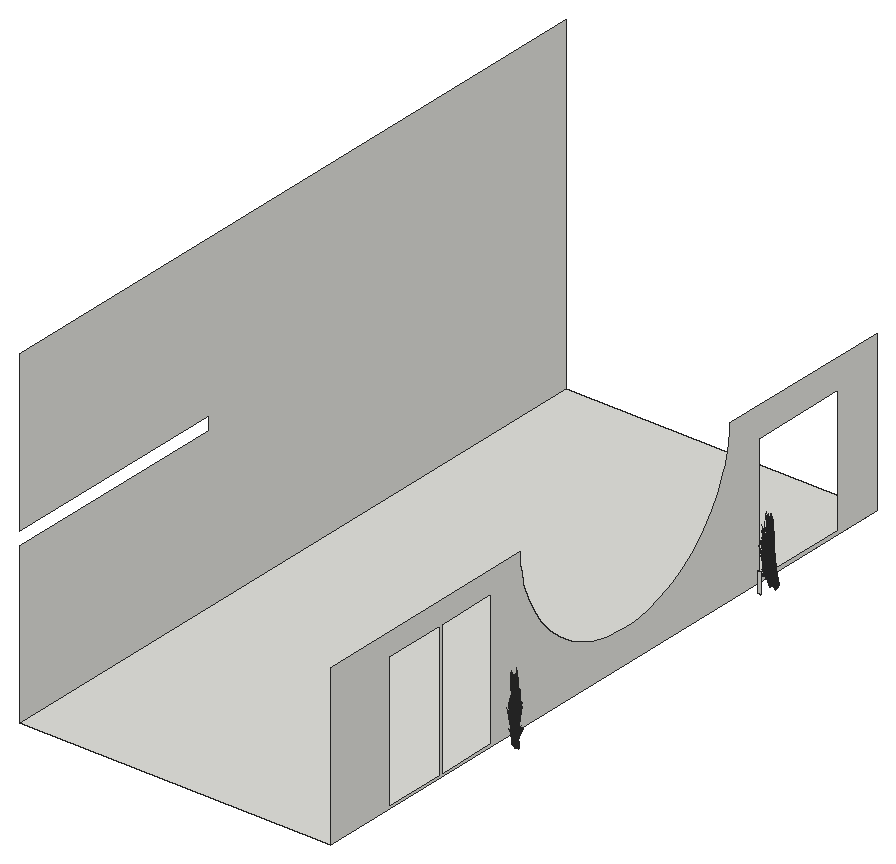
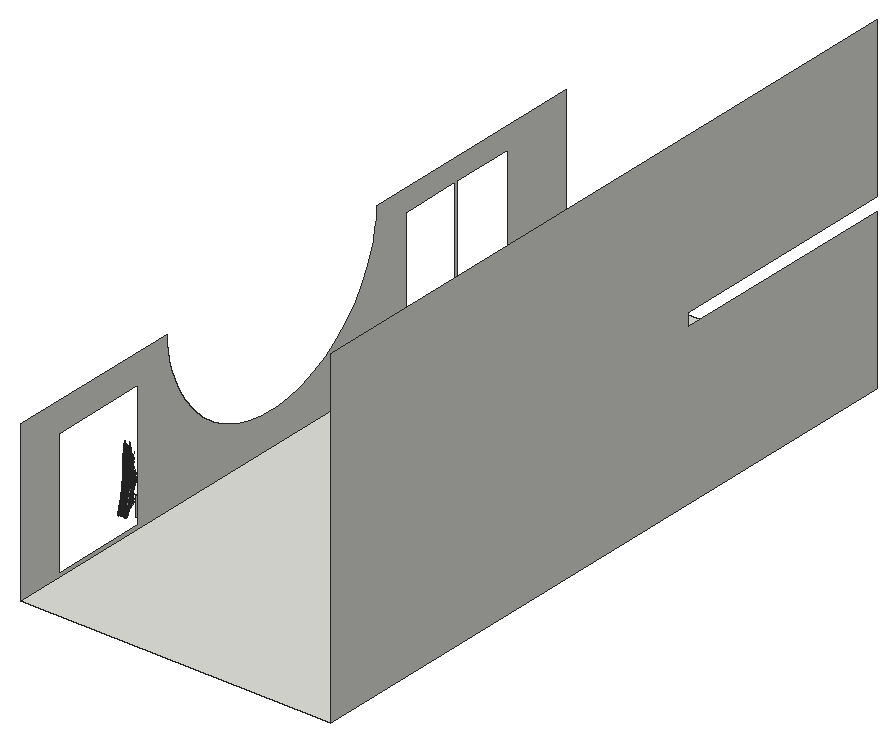
# SketchUp Ruby script. Lengths in inches.
U = 1.inch
M = Sketchup.active_model
def pt(a) = Geom::Point3d.new(a.map { |v| v * U })
def face(e, loops, mat)
  f = e.add_face(loops[0].map { |a| pt(a) })
  loops[1..].each { |l| e.add_face(l.map { |a| pt(a) }).erase! }
  f.material = f.back_material = mat if mat
  f
end
# faces: each face lists its corners as indices into pts; further lists are holes
def faces(e, pts, list, mat = nil) = list.each { |f| face(e, (f[0].is_a?(Array) ? f : [f]).map { |l| l.map { |i| pts[i] } }, mat) }
# xy, xz, yz: faces in a plane at the given z, y or x. An outline is a flat list of corners, or four numbers for a rectangle; further outlines are holes
def ring(l) = l.size == 4 ? [[l[0], l[1]], [l[2], l[1]], [l[2], l[3]], [l[0], l[3]]] : l.each_slice(2).to_a
def flat(e, list, mat, &to3) = list.each { |f| face(e, (f[0].is_a?(Array) ? f : [f]).map { |l| ring(l).map { |u, v| to3.(u, v) } }, mat) }
def xy(e, z, list, mat = nil) = flat(e, list, mat) { |x, y| [x, y, z] }
def xz(e, y, list, mat = nil) = flat(e, list, mat) { |x, z| [x, y, z] }
def yz(e, x, list, mat = nil) = flat(e, list, mat) { |y, z| [x, y, z] }
def lines(e, pts, list) = list.each { |a, b| e.add_line(pt(pts[a]), pt(pts[b])) }
# prism: a flat outline (further loops are holes) pulled along v
def prism(e, loops, v, mat = nil)
  f = face(e, loops, mat); d = Geom::Vector3d.new(v.map { |x| x * U })
  f.pushpull(f.normal.samedirection?(d) ? d.length : -d.length)
end
def box(e, o, s, mat = nil) = prism(e, [[o, [o[0] + s[0], o[1], o[2]], [o[0] + s[0], o[1] + s[1], o[2]], [o[0], o[1] + s[1], o[2]]]], [0, 0, s[2]], mat)
def at(x, y, z, deg = 0) = Geom::Transformation.translation(pt([x, y, z])) * Geom::Transformation.rotation(ORIGIN, Z_AXIS, deg.degrees)
def axes(o, x, y, z) = Geom::Transformation.new([*x, 0, *y, 0, *z, 0, *pt(o).to_a, 1])
def part(name) = M.definitions.add(name)
# library, detail: a bought-in or finely detailed component or shape, given as its bounding box
def library(name, o, s) = part(name).tap { |d| box(d.entities, o, s) }
def detail(e, o, s) = box(e.add_group.entities, o, s)
def put(e, d, t, mat = nil) = e.add_instance(d, t).tap { |i| i.material = mat if mat }
def group(e, t, mat = nil) = e.add_group.tap { |g| g.transformation = t; g.material = mat if mat }.entities
root = M.entities
M.materials.add("LightPink_Translucent").color = [144, 107, 117]
M.materials["LightPink_Translucent"].alpha = 0.75
c1 = part("blade")
p = [[2.15,0.21,22],[0,0.17,0],[0.09,0.45,0],[2.18,0.31,22],[2.29,0.31,22],[0.38,0.45,0],
  [2.48,0.24,33],[2.49,0.24,33],[2.48,0.22,33]]
faces(c1.entities,p,[[0,1,2,3],[4,5,2,3],[6,3,4,7],[8,0,3,6]])
c2 = part("seeds")
p = [[0.3,-0.1,1.38],[-0.01,-0.03,1.59],[-0.01,-0.03,0.03],[0.14,-0.07,-0.07],[0.29,-0.03,3],[0.15,0.01,3.11]]
faces(c2.entities,p,[[0,1,2,3],[1,0,4,5]],"LightPink_Translucent")
c3 = part("blade with seeds")
put(c3.entities,c1,at(0,0,0))
put(c3.entities,c2,axes([2.4,0.25,30.99],[1.5799,-0.05474,1.17369],[-0.12525,1.92788,0.29478],[-0.07173,-0.02425,1.56792]))
xy(root,618,[[39.57,167.5625,321.57,786.64]])
xz(root,361.54,[[330.57,618,333.57,636]])
xz(root,640.9,[[330.57,618,333.57,636]])
yz(root,39.57,[[167.5625,618,786.64,618,786.64,918,167.5625,918,167.5625,774,381.61,774,381.24,765.87,381.55,762,167.5625,762]])
yz(root,321.57,[[[167.5625,618,167.5625,762,381.51,762,381.51,761.73,382.09,755.37,382.45,750.85,382.53,750.46,382.63,749.39,385.28,737.31,385.54,736.1,385.57,736,385.87,734.67,390.92,720.47,397.71,707.02,406.14,694.53,416.0625,683.1875,427.33,673.18,439.76,664.67,453.17,657.78,467.33,652.62,482.02,649.28,497.02,647.81,501.22,647.92,512.08,648.23,526.98,650.53,541.46,654.68,555.3125,660.62,568.3125,668.24,580.25,677.43,590.95,688.05,600.23,699.93,607.94,712.87,613.98,726.68,614.22,727.97,617.96,740.22,620.52,755.07,620.84,762,786.64,762,786.64,618],[652.9,621,742.9,735],[233.15,620,291.15,742],[293.15,620,349.15,742]]])
put(root,c3,axes([334.28,650.62,623.6],[0.14639,-0.01056,1.71376],[-0.09712,0.45778,0.13857],[-0.20862,-0.02831,0.73262]))
put(root,c3,axes([334.71,650.19,624.71],[-0.35281,-0.01123,-0.71045],[0.0237,-0.47284,0.08574],[-0.14947,-0.0499,1.00501]))
put(root,c3,axes([334.43,650.31,622.31],[0.06891,0.12984,1.43002],[-0.15879,0.35293,-0.30754],[-0.16304,-0.08436,0.61141]))
put(root,c3,axes([334.55,649.89,623.6],[0.1311,0.08035,1.71376],[-0.27131,0.33708,0.13857],[-0.16909,-0.15206,0.73262]))
put(root,c3,axes([334.6,650.29,624.4],[-0.25628,0.30892,-0.51099],[-0.22444,-0.32634,-0.3958],[-0.13021,-0.047,0.97773]))
put(root,c3,axes([334.24,649.42,624.43],[0.02617,0.04654,1.77383],[-0.12614,0.41836,-0.16761],[-0.12775,0.00303,0.31391]))
put(root,c3,axes([334.53,649.15,624.4375],[-0.07594,-0.00329,1.74944],[-0.24177,0.32918,-0.27667],[-0.129,-0.06726,0.14031]))
put(root,c3,axes([334.73,649.97,624.76],[-0.0189,0.47427,-0.1216],[-0.35781,-0.01296,-0.67495],[-0.13781,-0.03295,1.02557]))
put(root,c3,axes([334.5,650,624.25],[-0.20082,-0.29199,-0.35414],[0.2293,-0.2764,0.4572],[-0.1165,-0.04206,0.87481]))
put(root,c3,axes([334.02,650.7,622.49],[0.22533,-0.03337,1.1486],[-0.14293,0.29403,0.84392],[-0.11135,-0.04411,0.25299]))
put(root,c3,axes([334.47,649.89,624.82],[0.29147,-0.34417,0.53763],[0.25138,0.3655,0.4433],[-0.13675,-0.06349,1.11249]))
put(root,c3,axes([334.6,649.89,624.45],[0.01777,-0.35463,0.0643],[0.26836,0.00972,0.50621],[-0.1028,-0.03711,0.77189]))
put(root,c3,axes([335.43,649.27,625.15],[-0.23555,0.44708,-0.13619],[-0.34112,-0.25757,-0.75594],[-0.11858,-0.12631,1.14864]))
put(root,c3,axes([334.79,650.15,624.78],[0.20082,0.29199,0.35414],[-0.2293,0.2764,-0.4572],[-0.1165,-0.04206,0.87481]))
put(root,c3,axes([335.33,649.64,624.71],[-0.30095,-0.22541,-0.71045],[0.21388,-0.395,0.08574],[-0.10904,-0.13459,1.00501]))
put(root,c3,axes([335.1875,649.65,624.4],[-0.34827,0.11086,-0.51099],[-0.06092,-0.41983,-0.3958],[-0.09354,-0.12031,0.97773]))
put(root,c3,axes([334.74,649.27,621.22],[-0.03419,0.06144,1.76342],[-0.3455,0.13246,-0.26939],[-0.08346,-0.12049,0.30037]))
put(root,c3,axes([334.52,649.5,621.85],[-0.10181,0.3808,-0.03893],[-0.31336,-0.11714,-0.17649],[-0.04758,-0.06228,0.58215]))
put(root,c3,axes([336.78,355.32,621.875],[0.12246,-0.09864,1.71376],[0.1031,0.45582,0.13857],[-0.19225,0.10302,0.73262]))
put(root,c3,axes([335.34,648.21,624.43],[-0.00658,0.0559,1.77383],[-0.32474,0.20287,-0.16761],[-0.09556,-0.1037,0.31391]))
put(root,c3,axes([334.99,649.02,622.31],[-0.02137,0.15256,1.43002],[-0.31245,0.12771,-0.30754],[-0.07303,-0.19719,0.61141]))
put(root,c3,axes([336.4,356.1,620.59],[0.12266,0.03828,1.43002],[0.07906,0.39104,-0.30754],[-0.16661,0.0732,0.61141]))
put(root,c3,axes([335.09,649.42,623.6],[0.08068,0.14973,1.71376],[-0.3728,0.12606,0.13857],[-0.08426,-0.23506,0.73262]))
put(root,c3,axes([335.22,649.34,624.25],[-0.05451,-0.37564,-0.35414],[0.31161,-0.09919,0.4572],[-0.0837,-0.10765,0.87481]))
put(root,c3,axes([337.49,354.85,621.34],[0.10032,-0.06746,1.77064],[0.0346,0.47103,0.13857],[-0.2173,0.0625,0.63284]))
put(root,c3,axes([334.35,651.24,622.1],[-0.44133,0,0],[0,-0.52122,-0.51607],[0,-0.11871,1.63711]))
put(root,c3,axes([335.41,649.65,624.78],[0.05451,0.37564,0.35414],[-0.31161,0.09919,-0.4572],[-0.0837,-0.10765,0.87481]))
put(root,c3,axes([336.41,355.16,622.72],[-0.05763,0.06055,1.74944],[0.0049,0.44239,-0.27667],[-0.13211,0.05753,0.14031]))
put(root,c3,axes([334.7,651.1,622.05],[-0.32829,0.39208,0.30756],[-0.32849,-0.38796,-0.36492],[-0.01146,-0.11134,1.64885]))
put(root,c3,axes([336.05,652.1875,623.05],[0.305,0.18805,1.51261],[-0.29879,0.40513,0.59816],[-0.13384,-0.24012,1.26806]))
put(root,c3,axes([334.88,648.78,622.49],[0.18411,0.16231,1.1486],[-0.26813,0.09757,0.84392],[-0.05737,-0.12474,0.25299]))
put(root,c3,axes([335.55,651.7,621.93],[-0.21202,-0.39143,-0.44739],[0.32115,-0.27564,0.21531],[-0.06861,-0.04843,1.43643]))
put(root,c3,axes([335.27,649.2,624.82],[0.39316,-0.11987,0.53763],[0.06823,0.47021,0.4433],[-0.09247,-0.13858,1.11249]))
put(root,c3,axes([335.77,355.61,622.71],[0.04504,0.01251,1.77383],[0.13934,0.41205,-0.16761],[-0.0922,0.10815,0.31391]))
put(root,c3,axes([336.79,355.11,622.68],[-0.09562,0.42421,-0.51099],[-0.32782,-0.1454,-0.3958],[-0.13199,0.0389,0.97773]))
put(root,c3,axes([335.36,649.3,624.45],[0.16041,-0.29625,0.0643],[0.22843,0.17248,0.50621],[-0.07385,-0.09498,0.77189]))
put(root,c3,axes([335.59,651.92,622.16],[0.09355,-0.55261,-0.23429],[0.44354,0.09633,0.51271],[-0.0775,-0.07631,1.5644]))
put(root,c3,axes([336.14,356.92,620.77],[0.14709,-0.21136,1.1486],[0.05804,0.3346,0.84392],[-0.1063,0.05991,0.25299]))
put(root,c3,axes([335.71,648.43,624.4375],[-0.05398,-0.06539,1.74944],[-0.36026,0.04145,-0.27667],[-0.0575,-0.15639,0.14031]))
put(root,c3,axes([334.45,650.89,621.74],[0,-0.46636,-0.49651],[0.39487,0,0],[0,-0.10622,1.57504]))
put(root,c3,axes([334.62,651.32,622.2],[0,0.46636,0.49651],[-0.39487,0,0],[0,-0.10622,1.57504]))
put(root,c3,axes([336.78,354.74,623.03],[0.17758,0.42229,-0.1216],[-0.31518,0.20752,-0.67495],[-0.13282,0.05572,1.02557]))
put(root,c3,axes([337.23,355.63,621.875],[0.08815,-0.14329,1.71376],[0.22258,0.38678,0.13857],[-0.15267,0.17614,0.73262]))
put(root,c3,axes([336.7,356.01,622.53],[-0.30722,0.06665,-0.35414],[-0.08112,-0.381,0.4572],[-0.08804,0.10234,0.87481]))
put(root,c3,axes([336.53,357.14,619.49],[0.04734,0.04659,1.76342],[0.08027,0.4317,-0.26939],[-0.10492,0.09206,0.30037]))
put(root,c3,axes([335.48,651.43,622.39],[-0.39748,-0.22252,-0.29095],[0.19139,-0.46966,-0.50002],[-0.01249,-0.11531,1.59708]))
put(root,c3,axes([336.74,355.92,622.73],[-0.08753,-0.42921,0.48003],[0.34336,-0.07449,0.3958],[-0.1012,0.10094,0.9933]))
put(root,c3,axes([335.31,650.95,621.82],[-0.14494,-0.47823,-0.69835],[0.41752,-0.17223,-0.18329],[-0.01602,-0.16194,1.54149]))
put(root,c3,axes([336.26,649.43,624.76],[-0.34538,0.21713,-0.1216],[-0.16972,-0.38536,-0.67495],[-0.04557,-0.16239,1.02557]))
put(root,c3,axes([335.96,649.45,624.4],[-0.34695,-0.11691,-0.51099],[0.11892,-0.40083,-0.3958],[-0.03181,-0.16138,0.97773]))
put(root,c3,axes([336.67,355.84,622.73],[-0.2423,-0.19613,0.0643],[0.14107,-0.2793,0.50621],[-0.07768,0.0903,0.77189]))
put(root,c3,axes([334.62,650.9,621.75],[0.24637,-0.29097,-0.30978],[0.24637,0.29097,0.30978],[0,-0.09372,1.38974]))
put(root,c3,axes([335.73,649.02,621.85],[-0.2439,0.26754,-0.03893],[-0.22348,-0.29302,-0.17649],[-0.01573,-0.08303,0.58215]))
put(root,c3,axes([337.16,355.98,621.875],[0.06572,-0.16029,1.71376],[0.27569,0.33172,0.13857],[-0.12437,0.20675,0.73262]))
put(root,c3,axes([338.74,650.62,623.1],[0.14639,-0.01056,1.71376],[-0.09712,0.45778,0.13857],[-0.20862,-0.02831,0.73262]))
put(root,c3,axes([336.09,649.53,624.71],[-0.16845,-0.3792,-0.71045],[0.34676,-0.21133,0.08574],[-0.03939,-0.18322,1.00501]))
put(root,c3,axes([336.95,356.05,622.68],[0.09067,0.42583,-0.51099],[-0.34336,0.07449,-0.3958],[-0.0984,0.11438,0.97773]))
put(root,c3,axes([336.42,356.82,622.72],[-0.00877,0.09229,1.74944],[0.24897,0.32105,-0.27667],[-0.06518,0.15182,0.14031]))
put(root,c3,axes([336.15,649.59,624.78],[-0.1064,0.35863,0.35414],[-0.31043,-0.1046,-0.4572],[-0.02846,-0.14439,0.87481]))
put(root,c3,axes([336.79,355.75,623.03],[0.32648,0.25715,-0.1216],[-0.18809,0.3724,-0.67495],[-0.09224,0.12945,1.02557]))
put(root,c3,axes([337.53,356.92,620.375],[-0.22066,0.46731,0],[-0.36918,-0.26061,-0.51607],[-0.08408,-0.05936,1.63711]))
put(root,c3,axes([335.8,648.6875,621.22],[-0.0592,0.0168,1.76342],[-0.32738,-0.18913,-0.26939],[0.00549,-0.15776,0.30037]))
put(root,c3,axes([336.25,356.86,623.65],[0.31145,0.12449,-0.06488],[-0.0958,0.38314,-0.29416],[-0.05094,0.05817,0.97024]))
put(root,c3,axes([336.95,355.78,623.05],[0.30722,-0.06665,0.35414],[0.08112,0.381,-0.4572],[-0.08804,0.10234,0.87481]))
put(root,c3,axes([336.12,649.21,624.25],[0.1064,-0.35863,-0.35414],[0.31043,0.1046,0.4572],[-0.02846,-0.14439,0.87481]))
put(root,c3,axes([335.6,651.14,622.09],[0.15345,0.52148,0.45755],[-0.43845,0.18134,0.17955],[0.00536,-0.09582,1.58856]))
put(root,c3,axes([335.53,651.08,621.93],[0.17124,-0.42022,-0.44739],[0.35581,0.20224,0.21531],[0,-0.09687,1.43643]))
put(root,c3,axes([337.125,357.6,620.59],[0.11138,-0.07357,1.43002],[0.27499,0.22183,-0.30754],[-0.08185,0.19194,0.61141]))
put(root,c3,axes([339.17,650.19,624.21],[-0.35281,-0.01123,-0.71045],[0.0237,-0.47284,0.08574],[-0.14947,-0.0499,1.00501]))
put(root,c3,axes([338.89,650.31,621.81],[0.06891,0.12984,1.43002],[-0.15879,0.35293,-0.30754],[-0.16304,-0.08436,0.61141]))
put(root,c3,axes([339.01,649.89,623.1],[0.1311,0.08035,1.71376],[-0.27131,0.33708,0.13857],[-0.16909,-0.15206,0.73262]))
put(root,c3,axes([337.24,356.79,622.73],[-0.25132,-0.3182,0.48003],[0.2669,-0.27442,0.3958],[-0.04636,0.14929,0.9933]))
put(root,c3,axes([337.15,356.76,622.73],[-0.29004,-0.02173,0.0643],[0.00795,-0.32812,0.50621],[-0.03035,0.12569,0.77189]))
put(root,c3,axes([336.25,649.26,624.45],[0.26007,-0.1585,0.0643],[0.12729,0.28902,0.50621],[-0.02512,-0.1274,0.77189]))
put(root,c3,axes([337.24,356.89,622.53],[-0.23881,0.24554,-0.35414],[-0.22606,-0.28036,0.4572],[-0.0344,0.14245,0.87481]))
put(root,c3,axes([339.8125,650.62,623.19],[0.14639,-0.01056,1.71376],[-0.09712,0.45778,0.13857],[-0.20862,-0.02831,0.73262]))
put(root,c3,axes([336.16,649.29,624.46],[0.34777,0.12192,0.48003],[-0.11892,0.40083,0.3958],[-0.0209,-0.15763,0.9933]))
put(root,c3,axes([335.74,651.29,622.16],[0.39767,0.22603,0.24065],[-0.19139,0.46966,0.50002],[0,-0.10827,1.60543]))
put(root,c3,axes([339.06,650.29,623.9],[-0.25628,0.30892,-0.51099],[-0.22444,-0.32634,-0.3958],[-0.13021,-0.047,0.97773]))
put(root,c3,axes([335.61,650.97,622.44],[-0.38326,0.02879,0.44739],[-0.03466,-0.47788,-0.21531],[0.06861,-0.04843,1.43643]))
put(root,c3,axes([338.46,356.15,620.06],[-0.23773,0.35053,-0.62353],[-0.29532,-0.31785,-0.16365],[-0.09526,0.08744,1.37633]))
put(root,c3,axes([336.39,357.76,622.71],[0.04004,-0.02816,1.77383],[0.33095,0.18728,-0.16761],[-0.00778,0.15594,0.31391]))
put(root,c3,axes([338.7,649.42,623.93],[0.02617,0.04654,1.77383],[-0.12614,0.41836,-0.16761],[-0.12775,0.00303,0.31391]))
put(root,c3,axes([338.99,649.15,623.9375],[-0.07594,-0.00329,1.74944],[-0.24177,0.32918,-0.27667],[-0.129,-0.06726,0.14031]))
put(root,c3,axes([338.625,355.96,620.46],[-0.34464,-0.37536,-0.25192],[0.29,-0.42149,0.5513],[-0.0928,0.04391,1.68216]))
put(root,c3,axes([335.25,649.58,622.1],[-0.22066,-0.46731,0],[0.36918,-0.26061,-0.51607],[0.08408,-0.05936,1.63711]))
put(root,c3,axes([337.4,356.63,623.34],[-0.00918,0.43138,-0.7886],[-0.38672,-0.02897,0.09517],[-0.04081,0.18275,1.11556]))
put(root,c3,axes([339.19,649.97,624.26],[-0.0189,0.47427,-0.1216],[-0.35781,-0.01296,-0.67495],[-0.13781,-0.03295,1.02557]))
put(root,c3,axes([338.96,650,623.75],[-0.20082,-0.29199,-0.35414],[0.2293,-0.2764,0.4572],[-0.1165,-0.04206,0.87481]))
put(root,c3,axes([337.39,357.84,620.77],[-0.00913,-0.2773,1.1486],[0.22824,0.19778,0.84392],[-0.04489,0.13217,0.25299]))
put(root,c3,axes([338.45,355.875,620.21],[-0.38326,0.02879,-0.44739],[-0.03466,-0.47788,0.21531],[-0.06861,0.04843,1.43643]))
put(root,c3,axes([336.17,648.45,622.49],[0.04528,0.27194,1.1486],[-0.25117,-0.15062,0.84392],[0.02703,-0.13924,0.25299]))
put(root,c3,axes([338.48,650.7,621.99],[0.22533,-0.03337,1.1486],[-0.14293,0.29403,0.84392],[-0.11135,-0.04411,0.25299]))
put(root,c3,axes([337.72,356.68,620.48],[0.33032,0.23318,0.49651],[-0.19744,0.41812,0],[-0.07523,-0.05311,1.57504]))
put(root,c3,axes([337.27,357.24,621.36],[0.00775,-0.24075,1.54345],[0.34877,0.12716,0.21329],[-0.03022,0.25658,0.72882]))
put(root,c3,axes([337.25,648.89,624.43],[-0.03584,0.03562,1.77383],[-0.35118,-0.12018,-0.16761],[-0.01271,-0.15545,0.31391]))
put(root,c3,axes([336.97,649.92,624.76],[-0.3879,-0.02311,-0.1216],[0.0106,-0.43749,-0.67495],[0.02694,-0.1685,1.02557]))
put(root,c3,axes([338.93,649.89,624.32],[0.29147,-0.34417,0.53763],[0.25138,0.3655,0.4433],[-0.13675,-0.06349,1.11249]))
put(root,c3,axes([338.85,357.11,620.02],[-0.33032,0.23318,-0.49651],[-0.19744,-0.41812,0],[-0.07523,0.05311,1.57504]))
put(root,c3,axes([338.875,356.98,620.19],[-0.21791,-0.46895,-0.05142],[0.36918,-0.26061,0.51607],[-0.09097,0.04465,1.6363]))
put(root,c3,axes([340.25,650.19,624.3],[-0.35281,-0.01123,-0.71045],[0.0237,-0.47284,0.08574],[-0.14947,-0.0499,1.00501]))
put(root,c3,axes([336.82,649.99,624.78],[-0.23881,0.24554,0.35414],[-0.22606,-0.28036,-0.4572],[0.0344,-0.14245,0.87481]))
put(root,c3,axes([335.68,650.87,622.39],[-0.04113,-0.53214,-0.29095],[0.42835,-0.03218,-0.50002],[0.07543,-0.07088,1.59708]))
put(root,c3,axes([339.97,650.31,621.91],[0.06891,0.12984,1.43002],[-0.15879,0.35293,-0.30754],[-0.16304,-0.08436,0.61141]))
put(root,c3,axes([337.48,356.77,623],[0.25266,0.31335,-0.5672],[-0.2669,0.27442,-0.43934],[-0.03844,0.15921,1.08528]))
put(root,c3,axes([336.71,649.76,624.4],[-0.25266,-0.31335,-0.51099],[0.2669,-0.27442,-0.3958],[0.03844,-0.15921,0.97773]))
put(root,c3,axes([338.78,356.93,620.03],[-0.32928,-0.11539,-0.30978],[0.08291,-0.40636,0.30978],[-0.06638,0.04686,1.38974]))
put(root,c3,axes([337.36,356.54,623.05],[0.23881,-0.24554,0.35414],[0.22606,0.28036,-0.4572],[-0.0344,0.14245,0.87481]))
put(root,c3,axes([340.09,649.89,623.19],[0.1311,0.08035,1.71376],[-0.27131,0.33708,0.13857],[-0.16909,-0.15206,0.73262]))
put(root,c3,axes([338.97,355.1875,620.84],[-0.00964,-0.43909,1.41272],[0.43635,0.11382,0.59816],[-0.1032,0.24027,1.3335]))
put(root,c3,axes([340.46,355.25,621.875],[0.12246,-0.09864,1.71376],[0.1031,0.45582,0.13857],[-0.19225,0.10302,0.73262]))
put(root,c3,axes([340.08,356.02,620.59],[0.12266,0.03828,1.43002],[0.07906,0.39104,-0.30754],[-0.16661,0.0732,0.61141]))
put(root,c3,axes([337.21,356.61,623.4],[0.3879,0.02311,-0.13498],[-0.0106,0.43749,-0.74919],[-0.02694,0.1685,1.13838]))
put(root,c3,axes([339.06,649.89,623.95],[0.01777,-0.35463,0.0643],[0.26836,0.00972,0.50621],[-0.1028,-0.03711,0.77189]))
put(root,c3,axes([335.63,649.69,621.75],[0.32928,0.11539,-0.30978],[-0.08291,0.40636,0.30978],[0.06638,-0.04686,1.38974]))
put(root,c3,axes([337.2,357.24,620.82],[0.32063,-0.08258,0.06507],[0.07371,0.33271,-0.86304],[-0.02033,0.16842,0.7736]))
put(root,c3,axes([338.72,355.75,620.67],[0.04113,0.53214,-0.29095],[-0.42835,0.03218,-0.50002],[-0.07543,0.07088,1.59708]))
put(root,c3,axes([339.89,649.27,624.65],[-0.23555,0.44708,-0.13619],[-0.34112,-0.25757,-0.75594],[-0.11858,-0.12631,1.14864]))
put(root,c3,axes([336.54,649.2,622.31],[-0.10032,0.0944,1.43002],[-0.30046,-0.16522,-0.30754],[0.05569,-0.20547,0.61141]))
put(root,c3,axes([340.13,650.29,624],[-0.25628,0.30892,-0.51099],[-0.22444,-0.32634,-0.3958],[-0.13021,-0.047,0.97773]))
put(root,c3,axes([339.25,650.15,624.28],[0.20082,0.29199,0.35414],[-0.2293,0.2764,-0.4572],[-0.1165,-0.04206,0.87481]))
put(root,c3,axes([337.76,356.32,621.875],[-0.00864,-0.17899,1.71376],[0.37441,0.11874,0.13857],[-0.02316,0.25508,0.73262]))
put(root,c3,axes([339.79,649.64,624.21],[-0.30095,-0.22541,-0.71045],[0.21388,-0.395,0.08574],[-0.10904,-0.13459,1.00501]))
put(root,c3,axes([335.55,649.51,621.74],[0.33032,-0.23318,-0.49651],[0.19744,0.41812,0],[0.07523,-0.05311,1.57504]))
put(root,c3,axes([339.65,649.65,623.9],[-0.34827,0.11086,-0.51099],[-0.06092,-0.41983,-0.3958],[-0.09354,-0.12031,0.97773]))
put(root,c3,axes([339.77,649.42,624.03],[0.02617,0.04654,1.77383],[-0.12614,0.41836,-0.16761],[-0.12775,0.00303,0.31391]))
put(root,c3,axes([341.15,650.62,623.58],[0.14639,-0.01056,1.71376],[-0.09712,0.45778,0.13857],[-0.20862,-0.02831,0.73262]))
put(root,c3,axes([339.2,649.27,620.72],[-0.03419,0.06144,1.76342],[-0.3455,0.13246,-0.26939],[-0.08346,-0.12049,0.30037]))
put(root,c3,axes([340.07,649.15,624.03],[-0.07594,-0.00329,1.74944],[-0.24177,0.32918,-0.27667],[-0.129,-0.06726,0.14031]))
put(root,c3,axes([340.09,355.09,622.72],[-0.05763,0.06055,1.74944],[0.0049,0.44239,-0.27667],[-0.13211,0.05753,0.14031]))
put(root,c3,axes([336.79,649.9,624.71],[0.00918,-0.43138,-0.71045],[0.38672,0.02897,0.08574],[0.04081,-0.18275,1.00501]))
put(root,c3,axes([340.27,649.97,624.35],[-0.0189,0.47427,-0.1216],[-0.35781,-0.01296,-0.67495],[-0.13781,-0.03295,1.02557]))
put(root,c3,axes([340.04,650,623.84],[-0.20082,-0.29199,-0.35414],[0.2293,-0.2764,0.4572],[-0.1165,-0.04206,0.87481]))
put(root,c3,axes([339.56,650.7,622.08],[0.22533,-0.03337,1.1486],[-0.14293,0.29403,0.84392],[-0.11135,-0.04411,0.25299]))
put(root,c3,axes([338.33,356.51,620.2],[-0.35581,-0.20937,0],[0.17124,-0.43505,0],[0,0,1.62707]))
put(root,c3,axes([339.44,355.53,622.71],[0.04504,0.01251,1.77383],[0.13934,0.41205,-0.16761],[-0.0922,0.10815,0.31391]))
put(root,c3,axes([339.15,357.04,620.375],[0.22066,0.46731,0],[-0.36918,0.26061,-0.51607],[-0.08408,0.05936,1.63711]))
put(root,c3,axes([340.47,355.03,622.68],[-0.09562,0.42421,-0.51099],[-0.32782,-0.1454,-0.3958],[-0.13199,0.0389,0.97773]))
put(root,c3,axes([338.98,649.5,621.35],[-0.10181,0.3808,-0.03893],[-0.31336,-0.11714,-0.17649],[-0.04758,-0.06228,0.58215]))
put(root,c3,axes([338.03,357.24,623.0625],[-0.34777,-0.12192,0.53283],[0.11892,-0.40083,0.43934],[0.0209,0.15763,1.10256]))
put(root,c3,axes([336.95,649.64,624.25],[0.23881,-0.24554,-0.35414],[0.22606,0.28036,0.4572],[0.0344,-0.14245,0.87481]))
put(root,c3,axes([337.9375,357.27,622.73],[-0.26007,0.1585,0.0643],[-0.12729,-0.28902,0.50621],[0.02512,0.1274,0.77189]))
put(root,c3,axes([339.8,648.21,623.93],[-0.00658,0.0559,1.77383],[-0.32474,0.20287,-0.16761],[-0.09556,-0.1037,0.31391]))
put(root,c3,axes([337.04,649.77,624.45],[0.29004,0.02173,0.0643],[-0.00795,0.32812,0.50621],[0.03035,-0.12569,0.77189]))
put(root,c3,axes([340.01,649.89,624.41],[0.29147,-0.34417,0.53763],[0.25138,0.3655,0.4433],[-0.13675,-0.06349,1.11249]))
put(root,c3,axes([339.45,649.02,621.81],[-0.02137,0.15256,1.43002],[-0.31245,0.12771,-0.30754],[-0.07303,-0.19719,0.61141]))
put(root,c3,axes([338.8,355.85,620.62],[0.26075,0.2802,0.1448],[-0.2175,0.31612,-0.41347],[-0.06054,0.04274,1.26744]))
put(root,c3,axes([339.55,649.42,623.1],[0.08068,0.14973,1.71376],[-0.3728,0.12606,0.13857],[-0.08426,-0.23506,0.73262]))
put(root,c3,axes([337.33,649.23,624.4375],[-0.00341,-0.09282,1.74944],[-0.28775,-0.26825,-0.27667],[0.04449,-0.16261,0.14031]))
put(root,c3,axes([335.94,650.46,621.78],[0.23773,-0.35053,-0.62353],[0.29532,0.31785,-0.16365],[0.09526,-0.08744,1.37633]))
put(root,c3,axes([336.95,649.74,624.46],[0.25132,0.3182,0.48003],[-0.2669,0.27442,0.3958],[0.04636,-0.14929,0.9933]))
put(root,c3,axes([338.79,355.64,620.72],[0.38326,-0.02879,0.44739],[0.03466,0.47788,-0.21531],[-0.06861,0.04843,1.43643]))
put(root,c3,axes([339.82,356.84,620.77],[0.14709,-0.21136,1.1486],[0.05804,0.3346,0.84392],[-0.1063,0.05991,0.25299]))
put(root,c3,axes([339.68,649.34,623.75],[-0.05451,-0.37564,-0.35414],[0.31161,-0.09919,0.4572],[-0.0837,-0.10765,0.87481]))
put(root,c3,axes([338.89,356.74,620.33],[0.44186,0.15158,0.30756],[-0.11054,0.54181,-0.36492],[-0.07313,0.06781,1.64885]))
put(root,c3,axes([338.8125,651.24,621.6],[-0.44133,0,0],[0,-0.52122,-0.51607],[0,-0.11871,1.63711]))
put(root,c3,axes([339.08,356.71,620.48],[0.33032,-0.23318,0.49651],[0.19744,0.41812,0],[-0.07523,0.05311,1.57504]))
put(root,c3,axes([340.46,354.66,623.03],[0.17758,0.42229,-0.1216],[-0.31518,0.20752,-0.67495],[-0.13282,0.05572,1.02557]))
put(root,c3,axes([340.91,355.55,621.875],[0.08815,-0.14329,1.71376],[0.22258,0.38678,0.13857],[-0.15267,0.17614,0.73262]))
put(root,c3,axes([340.38,355.93,622.53],[-0.30722,0.06665,-0.35414],[-0.08112,-0.381,0.4572],[-0.08804,0.10234,0.87481]))
put(root,c3,axes([337.99,357.18,619.49],[0.05712,-0.02538,1.76342],[0.34359,0.13968,-0.26939],[0.01005,0.15742,0.30037]))
put(root,c3,axes([340.14,649.89,624.05],[0.01777,-0.35463,0.0643],[0.26836,0.00972,0.50621],[-0.1028,-0.03711,0.77189]))
put(root,c3,axes([339.87,649.65,624.28],[0.05451,0.37564,0.35414],[-0.31161,0.09919,-0.4572],[-0.0837,-0.10765,0.87481]))
put(root,c3,axes([338.07,357.32,622.53],[-0.1064,0.35863,-0.35414],[-0.31043,-0.1046,0.4572],[0.02846,0.14439,0.87481]))
put(root,c3,axes([337.24,650.75,624.78],[-0.30722,0.06665,0.35414],[-0.08112,-0.381,-0.4572],[0.08804,-0.10234,0.87481]))
put(root,c3,axes([341.59,650.19,624.6875],[-0.35281,-0.01123,-0.71045],[0.0237,-0.47284,0.08574],[-0.14947,-0.0499,1.00501]))
put(root,c3,axes([340.21,357.06,619.49],[0.04734,0.04659,1.76342],[0.08027,0.4317,-0.26939],[-0.10492,0.09206,0.30037]))
put(root,c3,axes([339.16,651.1,621.55],[-0.32829,0.39208,0.30756],[-0.32849,-0.38796,-0.36492],[-0.01146,-0.11134,1.64885]))
put(root,c3,axes([340.97,649.27,624.75],[-0.23555,0.44708,-0.13619],[-0.34112,-0.25757,-0.75594],[-0.11858,-0.12631,1.14864]))
put(root,c3,axes([341.3,650.31,622.3],[0.06891,0.12984,1.43002],[-0.15879,0.35293,-0.30754],[-0.16304,-0.08436,0.61141]))
put(root,c3,axes([336.35,649.68,623.6],[-0.06572,0.16029,1.71376],[-0.27569,-0.33172,0.13857],[0.12437,-0.20675,0.73262]))
put(root,c3,axes([340.32,650.15,624.37],[0.20082,0.29199,0.35414],[-0.2293,0.2764,-0.4572],[-0.1165,-0.04206,0.87481]))
put(root,c3,axes([340.51,652.1875,622.55],[0.305,0.18805,1.51261],[-0.29879,0.40513,0.59816],[-0.13384,-0.24012,1.26806]))
put(root,c3,axes([341.43,649.89,623.58],[0.1311,0.08035,1.71376],[-0.27131,0.33708,0.13857],[-0.16909,-0.15206,0.73262]))
put(root,c3,axes([340.87,649.64,624.3],[-0.30095,-0.22541,-0.71045],[0.21388,-0.395,0.08574],[-0.10904,-0.13459,1.00501]))
put(root,c3,axes([339.34,648.78,621.99],[0.18411,0.16231,1.1486],[-0.26813,0.09757,0.84392],[-0.05737,-0.12474,0.25299]))
put(root,c3,axes([340.72,649.65,624],[-0.34827,0.11086,-0.51099],[-0.06092,-0.41983,-0.3958],[-0.09354,-0.12031,0.97773]))
put(root,c3,axes([340.42,355.85,622.73],[-0.08753,-0.42921,0.48003],[0.34336,-0.07449,0.3958],[-0.1012,0.10094,0.9933]))
put(root,c3,axes([340.01,651.7,621.43],[-0.21202,-0.39143,-0.44739],[0.32115,-0.27564,0.21531],[-0.06861,-0.04843,1.43643]))
put(root,c3,axes([338.875,355.54,620.21],[-0.17124,0.42022,-0.44739],[-0.35581,-0.20224,0.21531],[0,0.09687,1.43643]))
put(root,c3,axes([340.35,355.76,622.73],[-0.2423,-0.19613,0.0643],[0.14107,-0.2793,0.50621],[-0.07768,0.0903,0.77189]))
put(root,c3,axes([337.4,650.78,624.76],[-0.32648,-0.25715,-0.1216],[0.18809,-0.3724,-0.67495],[0.09224,-0.12945,1.02557]))
put(root,c3,axes([339.73,649.2,624.32],[0.39316,-0.11987,0.53763],[0.06823,0.47021,0.4433],[-0.09247,-0.13858,1.11249]))
put(root,c3,axes([340.28,649.27,620.81],[-0.03419,0.06144,1.76342],[-0.3455,0.13246,-0.26939],[-0.08346,-0.12049,0.30037]))
put(root,c3,axes([337.85,357.96,622.72],[0.04474,0.0751,1.74944],[0.36104,0.0295,-0.27667],[0.03631,0.16562,0.14031]))
put(root,c3,axes([339.55,355.28,620.47],[-0.2773,-0.3397,0.17642],[0.27945,-0.32949,0.35086],[-0.03063,0.06937,1.60407]))
put(root,c3,axes([341.47,650.29,624.39],[-0.25628,0.30892,-0.51099],[-0.22444,-0.32634,-0.3958],[-0.13021,-0.047,0.97773]))
put(root,c3,axes([338.82,355.3,620.29],[0,0.53934,-0.05637],[-0.44133,0,0],[0,0.01695,1.79368]))
put(root,c3,axes([340.84,355.91,621.875],[0.06572,-0.16029,1.71376],[0.27569,0.33172,0.13857],[-0.12437,0.20675,0.73262]))
put(root,c3,axes([339.82,649.3,623.95],[0.16041,-0.29625,0.0643],[0.22843,0.17248,0.50621],[-0.07385,-0.09498,0.77189]))
